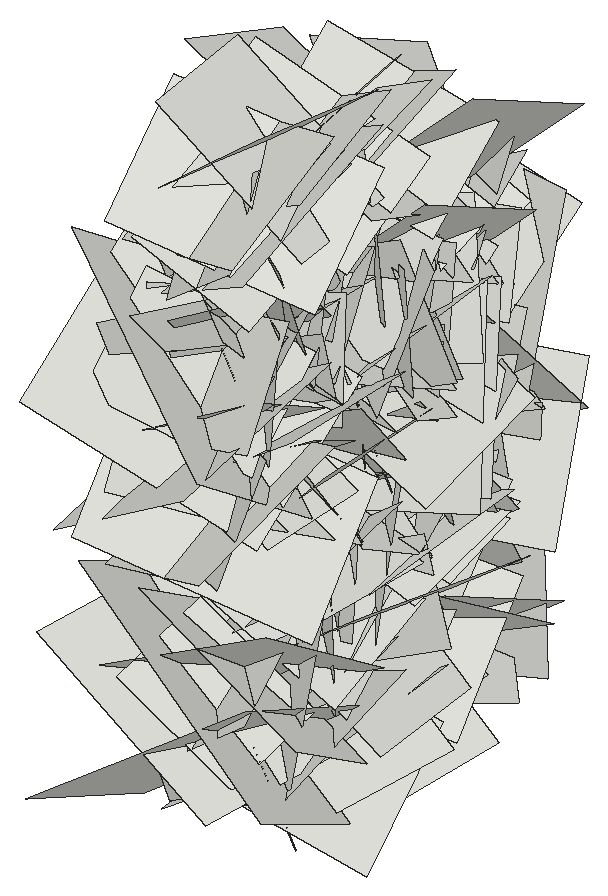
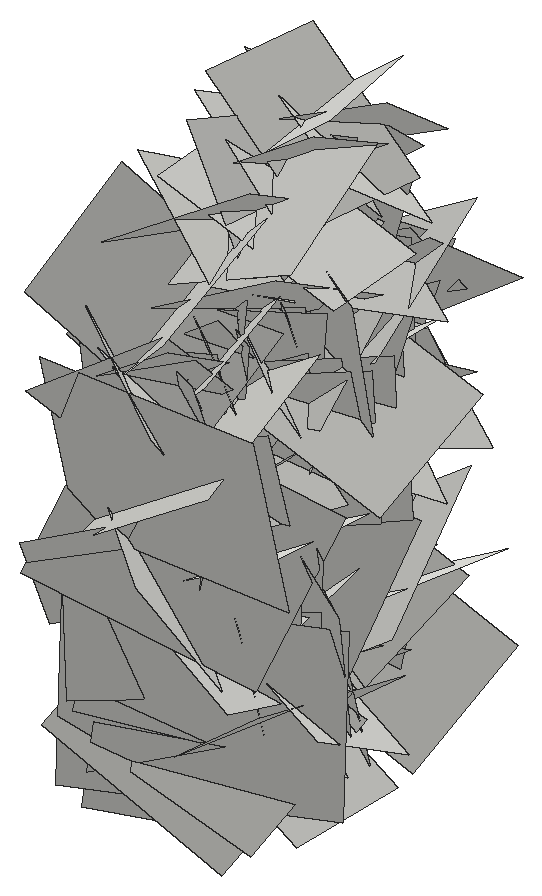
# SketchUp Ruby script. Lengths in inches.
U = 1.inch
M = Sketchup.active_model
def pt(a) = Geom::Point3d.new(a.map { |v| v * U })
def face(e, loops, mat)
  f = e.add_face(loops[0].map { |a| pt(a) })
  loops[1..].each { |l| e.add_face(l.map { |a| pt(a) }).erase! }
  f.material = f.back_material = mat if mat
  f
end
# faces: each face lists its corners as indices into pts; further lists are holes
def faces(e, pts, list, mat = nil) = list.each { |f| face(e, (f[0].is_a?(Array) ? f : [f]).map { |l| l.map { |i| pts[i] } }, mat) }
# xy, xz, yz: faces in a plane at the given z, y or x. An outline is a flat list of corners, or four numbers for a rectangle; further outlines are holes
def ring(l) = l.size == 4 ? [[l[0], l[1]], [l[2], l[1]], [l[2], l[3]], [l[0], l[3]]] : l.each_slice(2).to_a
def flat(e, list, mat, &to3) = list.each { |f| face(e, (f[0].is_a?(Array) ? f : [f]).map { |l| ring(l).map { |u, v| to3.(u, v) } }, mat) }
def xy(e, z, list, mat = nil) = flat(e, list, mat) { |x, y| [x, y, z] }
def xz(e, y, list, mat = nil) = flat(e, list, mat) { |x, z| [x, y, z] }
def yz(e, x, list, mat = nil) = flat(e, list, mat) { |y, z| [x, y, z] }
def lines(e, pts, list) = list.each { |a, b| e.add_line(pt(pts[a]), pt(pts[b])) }
# prism: a flat outline (further loops are holes) pulled along v
def prism(e, loops, v, mat = nil)
  f = face(e, loops, mat); d = Geom::Vector3d.new(v.map { |x| x * U })
  f.pushpull(f.normal.samedirection?(d) ? d.length : -d.length)
end
def box(e, o, s, mat = nil) = prism(e, [[o, [o[0] + s[0], o[1], o[2]], [o[0] + s[0], o[1] + s[1], o[2]], [o[0], o[1] + s[1], o[2]]]], [0, 0, s[2]], mat)
def at(x, y, z, deg = 0) = Geom::Transformation.translation(pt([x, y, z])) * Geom::Transformation.rotation(ORIGIN, Z_AXIS, deg.degrees)
def axes(o, x, y, z) = Geom::Transformation.new([*x, 0, *y, 0, *z, 0, *pt(o).to_a, 1])
def part(name) = M.definitions.add(name)
# library, detail: a bought-in or finely detailed component or shape, given as its bounding box
def library(name, o, s) = part(name).tap { |d| box(d.entities, o, s) }
def detail(e, o, s) = box(e.add_group.entities, o, s)
def put(e, d, t, mat = nil) = e.add_instance(d, t).tap { |i| i.material = mat if mat }
def group(e, t, mat = nil) = e.add_group.tap { |g| g.transformation = t; g.material = mat if mat }.entities
root = M.entities
c1 = part("Component\#6")
p = [[0.01,0,0],[0,3.24,4.54],[4.32,3.24,4.54],[4.33,0,0]]
faces(c1.entities,p,[[0,1,2,3]])
put(root,c1,axes([18.5,206.12,25.83],[-0.28838,0.48251,1.20317],[-0.13396,1.21365,-0.51529],[-1.36755,-0.22063,-0.20324]))
put(root,c1,axes([18.5,205.05,35.75],[-0.23328,1.34713,-0.22992],[-0.05022,-0.24027,-1.36238],[-1.44774,-0.20874,0.08431]))
put(root,c1,axes([18.85,214.11,35.21],[-0.07772,-0.27644,-1.33377],[-0.91911,-1.02064,0.2592],[-1.11351,0.86175,-0.12086]))
put(root,c1,axes([18.5,205.51,24.88],[-0.13882,1.11155,0.63897],[-0.19603,0.6192,-1.11507],[-1.34484,-0.205,0.09658]))
put(root,c1,axes([18.5,213.57,27.56],[0.01798,0.03957,-1.39555],[-0.22262,-1.3797,-0.04168],[-1.46303,0.21042,-0.01081]))
put(root,c1,axes([18.5,211.92,20.51],[-0.20622,-1.25394,-0.15944],[0.06822,-0.17093,1.26581],[-1.33814,0.18453,0.0891]))
put(root,c1,axes([18.5,204.65,33.57],[-0.11682,0.36237,1.1463],[-0.15256,1.13885,-0.37385],[-1.26518,-0.17079,-0.06076]))
put(root,c1,axes([18.5,205.46,24.09],[-0.08024,0.04196,1.34674],[0.06239,1.34768,-0.03868],[-1.42687,0.05657,-0.07742]))
put(root,c1,axes([18.5,205.63,39.17],[-0.17317,1.06099,0.10432],[-0.22006,0.07185,-1.05594],[-1.10844,-0.18002,0.19334]))
put(root,c1,axes([18.5,205.99,22.98],[-0.14358,-1.11124,-0.06865],[-0.09474,-0.05808,1.11649],[-1.17635,0.14031,-0.08154]))
put(root,c1,axes([18.5,203.71,22.72],[0.0324,0.32539,1.27516],[-0.00551,1.27553,-0.32536],[-1.39498,0.00251,0.0309]))
put(root,c1,axes([18.5,211.85,35.53],[-0.11979,-0.95717,-0.48165],[-0.13908,-0.46832,0.96146],[-1.12727,0.15949,-0.06744]))
put(root,c1,axes([18.5,211.375,32.78],[0.08242,0.8278,-0.94283],[-0.12426,-0.93571,-0.83122],[-1.32412,0.13934,0.01932]))
put(root,c1,axes([18.5,213.71,29.11],[0.07729,-1.24842,0.49404],[0.03127,0.49613,1.24937],[-1.42283,-0.05691,0.0543]))
put(root,c1,axes([18.5,208.94,26.04],[0.1299,1.02121,-0.60997],[-0.25035,-0.5801,-1.01865],[-1.23578,0.22487,0.14225]))
put(root,c1,axes([18.5,209.74,33.23],[-0.15201,0.07034,-1.21602],[0.20156,-1.20811,-0.09231],[-1.2753,-0.19933,0.13035]))
put(root,c1,axes([18.5,204.59,30.02],[0.04301,-1.09683,0.72238],[0.12053,0.72294,1.0913],[-1.38692,0.02882,0.11724]))
put(root,c1,axes([18.5,201.85,37.73],[0.10519,1.13817,0.58904],[0.00109,0.59073,-1.14161],[-1.35845,0.08861,0.0447]))
put(root,c1,axes([18.5,213.06,27.02],[0.109,-1.16412,-0.17966],[-0.1638,-0.19212,1.15639],[-1.23778,-0.07709,-0.16885]))
put(root,c1,axes([18.5,201.95,25.76],[-0.02109,1.10253,-0.4508],[0.04504,-0.44992,-1.10225],[-1.2618,-0.03449,-0.03181]))
put(root,c1,axes([18.5,213.59,29.33],[-0.10669,0.07311,-1.12569],[0.06812,-1.12796,-0.079],[-1.19381,-0.0709,0.09609]))
put(root,c1,axes([18.5,208.81,31.45],[0.04602,0.84125,-1.04893],[0.18208,-1.04435,-0.83047],[-1.4136,-0.10713,-0.14111]))
put(root,c1,axes([18.5,210.75,36.02],[0.14272,-1.0645,0.43866],[-0.22696,0.41079,1.0626],[-1.19913,-0.20445,-0.14891]))
put(root,c1,axes([18.5,205.38,23.16],[-0.04798,1.09948,0.05597],[-0.01409,0.05547,-1.10036],[-1.16688,-0.04588,0.01099]))
put(root,c1,axes([14.53,202.49,32.61],[-0.11645,-0.17214,0.59947],[-0.01233,0.60916,0.17278],[0.661,-0.01896,0.10883]))
put(root,c1,axes([18.5,206.95,24.98],[-0.09414,0.39654,1.07266],[0.12922,1.07305,-0.38659],[-1.20532,0.08407,-0.12522]))
put(root,c1,axes([18.5,211.99,33.59],[0.13241,-0.25962,-1.28668],[0.09489,-1.2878,0.26854],[-1.38813,-0.1128,-0.10438]))
put(root,c1,axes([18.5,206.8125,26.89],[0.15204,1.11982,0.24611],[-0.19339,0.26716,-1.10927],[-1.19986,0.09884,0.20998]))
put(root,c1,axes([18.5,206.55,33.15],[-0.00164,-0.95203,-0.71322],[0.09471,-0.7113,0.94927],[-1.25737,-0.05234,0.07244]))
put(root,c1,axes([14.53,210.56,30.82],[-0.08988,0.23539,0.56706],[0.00516,0.57268,-0.23699],[0.65079,0.02797,0.0802]))
put(root,c1,axes([14.53,206,31.6],[-0.1462,-0.08624,0.716],[-0.07336,0.72719,0.07426],[0.76092,0.05354,0.14472]))
put(root,c1,axes([18.5,207.91,30.98],[0.03881,-0.77727,0.6188],[-0.26695,0.59174,0.75817],[-1.01873,-0.18467,-0.1751]))
put(root,c1,axes([18.5,205.46,33.43],[-0.14097,0.63084,0.7943],[0.06243,0.80455,-0.62912],[-1.07339,-0.03606,-0.14091]))
put(root,c1,axes([18.5,212.99,32.26],[-0.05541,-0.21084,-0.92918],[-0.15034,-0.91849,0.21639],[-0.99872,0.14996,0.01898]))
put(root,c1,axes([18.5,208.01,36.375],[0.10923,0.38133,-1.06486],[-0.05778,-1.06635,-0.38714],[-1.19755,0.08623,-0.07845]))
put(root,c1,axes([18.5,206.07,20.81],[0.31441,-1.20333,0.63493],[0.01893,0.65323,1.22967],[-1.44208,-0.25378,0.15457]))
put(root,c1,axes([18.5,199.54,32.72],[0.14681,1.15124,0.44909],[0.05729,0.44582,-1.15954],[-1.30862,0.14867,-0.00039]))
put(root,c1,axes([18.5,211.43,33.78],[0.23599,-0.36182,-1.29322],[0.09706,-1.30373,0.38052],[-1.42014,-0.14923,-0.18889]))
put(root,c1,axes([18.5,212.85,24.81],[0.10314,-0.72888,-0.73382],[-0.20394,-0.73695,0.70648],[-1.07722,0.06973,-0.20401]))
put(root,c1,axes([18.5,211.63,27.44],[-0.13698,0.50835,-0.7639],[-0.02564,-0.77306,-0.51036],[-0.97231,-0.05123,0.12108]))
put(root,c1,axes([14.53,207.84,29.22],[-0.13906,-0.51177,-0.49755],[0.00544,-0.50655,0.51967],[0.75658,-0.09042,-0.09518]))
put(root,c1,axes([14.53,210.37,37.54],[-0.0852,-0.7988,-0.26142],[-0.21653,-0.23617,0.78446],[0.8642,-0.13792,0.17078]))
put(root,c1,axes([18.5,212.41,27.7],[-0.11035,-0.46639,-0.85158],[0.0233,-0.85737,0.46687],[-1.02892,0.03061,0.1019]))
put(root,c1,axes([18.5,209.77,25.57],[0.04769,1.02209,-0.46416],[0.05126,-0.46587,-1.02116],[-1.18879,0.02092,-0.06265]))
put(root,c1,axes([14.53,211.4,20.36],[-0.11841,0.02386,0.67628],[0.07272,0.6823,-0.01274],[0.7136,-0.06557,0.11352]))
put(root,c1,axes([14.53,208.95,27.68],[-0.1117,0.11156,-0.75397],[-0.06454,-0.75994,-0.10393],[0.80532,-0.04543,-0.11291]))
put(root,c1,axes([14.53,203.96,20.97],[0.02025,-0.24988,0.58047],[-0.03388,0.57961,0.25056],[0.66903,0.03691,-0.00488]))
put(root,c1,axes([14.53,202.42,34.22],[-0.03507,0.56649,-0.26791],[0.06705,-0.26389,-0.56581],[0.66085,0.05684,0.04319]))
put(root,c1,axes([18.5,211.47,22.62],[0.20513,-1.22241,0.07319],[0.04122,0.08019,1.23659],[-1.29742,-0.19072,0.05085]))
put(root,c1,axes([18.5,206.36,33.23],[0.09168,1.1059,0.20164],[0.04784,0.19866,-1.1089],[-1.19063,0.09314,-0.02903]))
put(root,c1,axes([18.5,205.67,24.52],[-0.15369,0.87531,0.08009],[0.01982,0.08422,-0.88666],[-0.9315,-0.14262,-0.03208]))
put(root,c1,axes([18.5,207.21,30.03],[0.00943,-1.01637,-0.0193],[0.00822,-0.01923,1.01638],[-1.07752,-0.00904,0.00758]))
put(root,c1,axes([14.53,204.95,35.05],[0.03568,0.1968,-0.61743],[-0.04358,-0.61637,-0.1987],[0.68554,-0.04943,0.01951]))
put(root,c1,axes([14.53,212.36,26.625],[-0.06935,-0.64087,-0.11796],[0.11905,-0.12787,0.63241],[0.68039,-0.04294,-0.12268]))
put(root,c1,axes([14.53,206.625,39.5],[-0.00312,0.09172,-0.66161],[0.00201,-0.66161,-0.09173],[0.70801,0.00228,-0.00265]))
put(root,c1,axes([14.53,204.22,36.67],[0.08595,0.41822,-0.43473],[-0.01861,-0.43682,-0.42351],[0.63917,-0.06896,0.04613]))
put(root,c1,axes([14.53,202.23,33.91],[0.02493,0.60398,0.49928],[-0.17768,0.49182,-0.58706],[0.81142,0.08914,-0.14389]))
put(root,c1,axes([14.53,200.85,29.625],[-0.04324,0.39016,0.69087],[-0.10275,0.68414,-0.39209],[0.83473,0.10443,-0.01247]))
put(root,c1,axes([14.53,212.78,35.18],[-0.06835,-0.19577,-0.64021],[0.13077,-0.63563,0.18195],[0.69749,0.09999,-0.09685]))
put(root,c1,axes([14.53,211.1,35.2],[0.07899,0.5337,0.27791],[0.02897,0.27674,-0.53878],[0.63716,-0.07875,-0.00996]))
put(root,c1,axes([18.5,202.75,27.49],[0.17368,0.85862,-0.51485],[-0.1903,-0.48804,-0.87105],[-1.04401,0.2318,0.07312]))
put(root,c1,axes([14.53,206.77,29.69],[0.13468,0.0618,0.68245],[-0.14259,0.68282,-0.03679],[0.71222,0.12502,-0.13642]))
put(root,c1,axes([18.5,204.74,34.65],[-0.08046,-0.48471,-0.63269],[-0.12911,-0.62103,0.49039],[-0.83492,0.14274,-0.01486]))
put(root,c1,axes([18.5,210.61,30.96],[-0.02538,-1.03384,0.49264],[0.2847,0.47394,1.00764],[-1.18007,0.13657,0.23251]))
put(root,c1,axes([18.5,212.48,33.12],[-0.02538,-1.03384,0.49264],[0.2847,0.47394,1.00764],[-1.18007,0.13657,0.23251]))
put(root,c1,axes([18.5,201.41,38.375],[0.12316,0.77538,0.57304],[-0.12545,0.58429,-0.76661],[-1.01427,0.02189,0.1644]))
put(root,c1,axes([14.53,207.11,31.75],[-0.23783,0.22127,0.93353],[-0.03566,0.95632,-0.23476],[1.01634,0.08533,0.21022]))
put(root,c1,axes([18.5,210.23,35.31],[-0.06568,0.00099,-0.81141],[-0.08224,-0.81005,0.00494],[-0.85616,0.07773,0.06177]))
put(root,c1,axes([14.53,204.33,34.72],[-0.02793,-0.28222,0.66343],[0.05268,0.66158,0.28341],[0.7624,-0.05605,0.00473]))
put(root,c1,axes([14.53,209.27,26.93],[0.01951,-0.6006,0.29742],[0.06663,0.29777,0.59742],[0.70729,-0.01148,-0.06448]))
put(root,c1,axes([18.5,205.35,34.65],[-0.12302,0.37909,0.72016],[0.00858,0.72795,-0.38188],[-0.86263,-0.04682,-0.1065]))
put(root,c1,axes([18.5,204.65,32.19],[-0.14144,0.68446,-0.34907],[-0.03425,-0.35898,-0.69154],[-0.81371,-0.10387,0.08978]))
put(root,c1,axes([14.53,205,37.54],[0.1597,-0.46751,-0.41946],[-0.05532,-0.43919,0.47075],[0.66349,0.07592,0.14021]))
put(root,c1,axes([14.53,211.91,37.97],[-0.10192,-0.72839,-0.40458],[-0.00784,-0.4065,0.73361],[0.88316,-0.08767,-0.04018]))
put(root,c1,axes([14.53,207.4,37.82],[-0.14382,-0.92009,0.02073],[-0.06912,0.03051,0.92748],[0.97309,-0.13382,0.06894]))
put(root,c1,axes([18.5,206.58,28.49],[-0.01093,-0.51913,0.63451],[-0.10311,0.63085,0.51456],[-0.86287,-0.06881,-0.06953]))
put(root,c1,axes([14.53,201.89,25.36],[0.12511,0.60489,0.30184],[-0.04372,0.31228,-0.60968],[0.71524,-0.08672,-0.09007]))
put(root,c1,axes([14.53,209.37,33.75],[-0.00852,0.3462,-0.76666],[-0.09329,-0.76284,-0.34355],[0.88678,-0.07692,-0.04351]))
put(root,c1,axes([18.5,210.92,34.25],[-0.13403,0.53039,0.57824],[0.04314,0.58935,-0.53168],[-0.83061,-0.05497,-0.12092]))
put(root,c1,axes([14.53,209.14,33.82],[0.16184,0.36707,0.52708],[-0.01835,0.54392,-0.37378],[0.68059,-0.07262,-0.13541]))
put(root,c1,axes([18.5,204.07,39.0625],[0.02986,0.79051,0.40956],[-0.00815,0.40997,-0.79076],[-0.94369,0.02147,0.01979]))
put(root,c1,axes([14.53,207.43,34.16],[0.11276,0.04323,0.70746],[-0.03845,0.71477,-0.03823],[0.75032,0.03013,-0.10828]))
put(root,c1,axes([18.5,200.125,30.08],[0.25415,0.9144,0.59243],[0.00684,0.60541,-0.93704],[-1.1549,0.20481,0.12483]))
put(root,c1,axes([18.5,209.72,22.08],[0.18138,-0.91546,-0.54155],[0.07402,-0.53767,0.93095],[-1.12504,-0.18297,-0.02606]))
put(root,c1,axes([18.5,208.86,27.22],[0.22907,0.58895,0.94038],[0.09031,0.94642,-0.61231],[-1.17269,0.18793,0.13653]))
put(root,c1,axes([18.5,209.27,26.87],[-0.02942,-0.98917,0.00062],[0.2303,-0.00549,0.9654],[-1.02292,0.02721,0.21733]))
put(root,c1,axes([14.53,202.89,32.22],[-0.0211,0.0618,0.84202],[-0.01452,0.84212,-0.06213],[0.89482,0.01512,0.01885]))
put(root,c1,axes([18.5,210.17,27.25],[-0.0389,-0.19659,0.74237],[-0.03773,0.74285,0.19496],[-0.81316,-0.02506,-0.04456]))
put(root,c1,axes([18.5,209.1,25.86],[0.06992,-0.92649,-0.30548],[0.11921,-0.29692,0.92479],[-1.02719,-0.09753,0.08653]))
put(root,c1,axes([14.53,209.1,25.86],[-0.06992,-0.92649,-0.30548],[-0.11921,-0.29692,0.92479],[1.02719,-0.09753,0.08653]))
put(root,c1,axes([14.53,210.17,27.25],[0.0389,-0.19659,0.74237],[0.03773,0.74285,0.19496],[0.81316,-0.02506,-0.04456]))
put(root,c1,axes([18.5,202.89,32.22],[0.0211,0.0618,0.84202],[0.01452,0.84212,-0.06213],[-0.89482,0.01512,0.01885]))
put(root,c1,axes([14.53,209.27,26.87],[0.02942,-0.98917,0.00062],[-0.2303,-0.00549,0.9654],[1.02292,0.02721,0.21733]))
put(root,c1,axes([14.53,208.86,27.22],[-0.22907,0.58895,0.94038],[-0.09031,0.94642,-0.61231],[1.17269,0.18793,0.13653]))
put(root,c1,axes([14.53,209.72,22.08],[-0.18138,-0.91546,-0.54155],[-0.07402,-0.53767,0.93095],[1.12504,-0.18297,-0.02606]))
put(root,c1,axes([14.53,200.125,30.08],[-0.25415,0.9144,0.59243],[-0.00684,0.60541,-0.93704],[1.1549,0.20481,0.12483]))
put(root,c1,axes([18.5,207.43,34.16],[-0.11276,0.04323,0.70746],[0.03845,0.71477,-0.03823],[-0.75032,0.03013,-0.10828]))
put(root,c1,axes([14.53,204.07,39.0625],[-0.02986,0.79051,0.40956],[0.00815,0.40997,-0.79076],[0.94369,0.02147,0.01979]))
put(root,c1,axes([18.5,209.14,33.82],[-0.16184,0.36707,0.52708],[0.01835,0.54392,-0.37378],[-0.68059,-0.07262,-0.13541]))
put(root,c1,axes([14.53,210.92,34.25],[0.13403,0.53039,0.57824],[-0.04314,0.58935,-0.53168],[0.83061,-0.05497,-0.12092]))
put(root,c1,axes([18.5,209.37,33.75],[0.00852,0.3462,-0.76666],[0.09329,-0.76284,-0.34355],[-0.88678,-0.07692,-0.04351]))
put(root,c1,axes([18.5,201.89,25.36],[-0.12511,0.60489,0.30184],[0.04372,0.31228,-0.60968],[-0.71524,-0.08672,-0.09007]))
put(root,c1,axes([14.53,206.58,28.49],[0.01093,-0.51913,0.63451],[0.10311,0.63085,0.51456],[0.86287,-0.06881,-0.06953]))
put(root,c1,axes([18.5,207.4,37.82],[0.14382,-0.92009,0.02073],[0.06912,0.03051,0.92748],[-0.97309,-0.13382,0.06894]))
put(root,c1,axes([18.5,211.91,37.97],[0.10192,-0.72839,-0.40458],[0.00784,-0.4065,0.73361],[-0.88316,-0.08767,-0.04018]))
put(root,c1,axes([18.5,205,37.54],[-0.1597,-0.46751,-0.41946],[0.05532,-0.43919,0.47075],[-0.66349,0.07592,0.14021]))
put(root,c1,axes([14.53,204.65,32.19],[0.14144,0.68446,-0.34907],[0.03425,-0.35898,-0.69154],[0.81371,-0.10387,0.08978]))
put(root,c1,axes([14.53,205.35,34.65],[0.12302,0.37909,0.72016],[-0.00858,0.72795,-0.38188],[0.86263,-0.04682,-0.1065]))
put(root,c1,axes([18.5,209.27,26.93],[-0.01951,-0.6006,0.29742],[-0.06663,0.29777,0.59742],[-0.70729,-0.01148,-0.06448]))
put(root,c1,axes([18.5,204.33,34.72],[0.02793,-0.28222,0.66343],[-0.05268,0.66158,0.28341],[-0.7624,-0.05605,0.00473]))
put(root,c1,axes([14.53,210.23,35.31],[0.06568,0.00099,-0.81141],[0.08224,-0.81005,0.00494],[0.85616,0.07773,0.06177]))
put(root,c1,axes([18.5,207.11,31.75],[0.23783,0.22127,0.93353],[0.03566,0.95632,-0.23476],[-1.01634,0.08533,0.21022]))
put(root,c1,axes([14.53,201.41,38.375],[-0.12316,0.77538,0.57304],[0.12545,0.58429,-0.76661],[1.01427,0.02189,0.1644]))
put(root,c1,axes([14.53,210.61,30.96],[0.02538,-1.03384,0.49264],[-0.2847,0.47394,1.00764],[1.18007,0.13657,0.23251]))
put(root,c1,axes([14.53,212.48,33.12],[0.02538,-1.03384,0.49264],[-0.2847,0.47394,1.00764],[1.18007,0.13657,0.23251]))
put(root,c1,axes([14.53,204.74,34.65],[0.08046,-0.48471,-0.63269],[0.12911,-0.62103,0.49039],[0.83492,0.14274,-0.01486]))
put(root,c1,axes([18.5,206.77,29.69],[-0.13468,0.0618,0.68245],[0.14259,0.68282,-0.03679],[-0.71222,0.12502,-0.13642]))
put(root,c1,axes([14.53,202.75,27.49],[-0.17368,0.85862,-0.51485],[0.1903,-0.48804,-0.87105],[1.04401,0.2318,0.07312]))
put(root,c1,axes([18.5,211.1,35.2],[-0.07899,0.5337,0.27791],[-0.02897,0.27674,-0.53878],[-0.63716,-0.07875,-0.00996]))
put(root,c1,axes([18.5,212.78,35.18],[0.06835,-0.19577,-0.64021],[-0.13077,-0.63563,0.18195],[-0.69749,0.09999,-0.09685]))
put(root,c1,axes([18.5,200.85,29.625],[0.04324,0.39016,0.69087],[0.10275,0.68414,-0.39209],[-0.83473,0.10443,-0.01247]))
put(root,c1,axes([18.5,202.23,33.91],[-0.02493,0.60398,0.49928],[0.17768,0.49182,-0.58706],[-0.81142,0.08914,-0.14389]))
put(root,c1,axes([18.5,204.22,36.67],[-0.08595,0.41822,-0.43473],[0.01861,-0.43682,-0.42351],[-0.63917,-0.06896,0.04613]))
put(root,c1,axes([18.5,206.625,39.5],[0.00312,0.09172,-0.66161],[-0.00201,-0.66161,-0.09173],[-0.70801,0.00228,-0.00265]))
put(root,c1,axes([18.5,212.36,26.625],[0.06935,-0.64087,-0.11796],[-0.11905,-0.12787,0.63241],[-0.68039,-0.04294,-0.12268]))
put(root,c1,axes([18.5,204.95,35.05],[-0.03568,0.1968,-0.61743],[0.04358,-0.61637,-0.1987],[-0.68554,-0.04943,0.01951]))
put(root,c1,axes([14.53,207.21,30.03],[-0.00943,-1.01637,-0.0193],[-0.00822,-0.01923,1.01638],[1.07752,-0.00904,0.00758]))
put(root,c1,axes([14.53,205.67,24.52],[0.15369,0.87531,0.08009],[-0.01982,0.08422,-0.88666],[0.9315,-0.14262,-0.03208]))
put(root,c1,axes([14.53,206.36,33.23],[-0.09168,1.1059,0.20164],[-0.04784,0.19866,-1.1089],[1.19063,0.09314,-0.02903]))
put(root,c1,axes([14.53,211.47,22.62],[-0.20513,-1.22241,0.07319],[-0.04122,0.08019,1.23659],[1.29742,-0.19072,0.05085]))
put(root,c1,axes([18.5,202.42,34.22],[0.03507,0.56649,-0.26791],[-0.06705,-0.26389,-0.56581],[-0.66085,0.05684,0.04319]))
put(root,c1,axes([18.5,203.96,20.97],[-0.02025,-0.24988,0.58047],[0.03388,0.57961,0.25056],[-0.66903,0.03691,-0.00488]))
put(root,c1,axes([18.5,208.95,27.68],[0.1117,0.11156,-0.75397],[0.06454,-0.75994,-0.10393],[-0.80532,-0.04543,-0.11291]))
